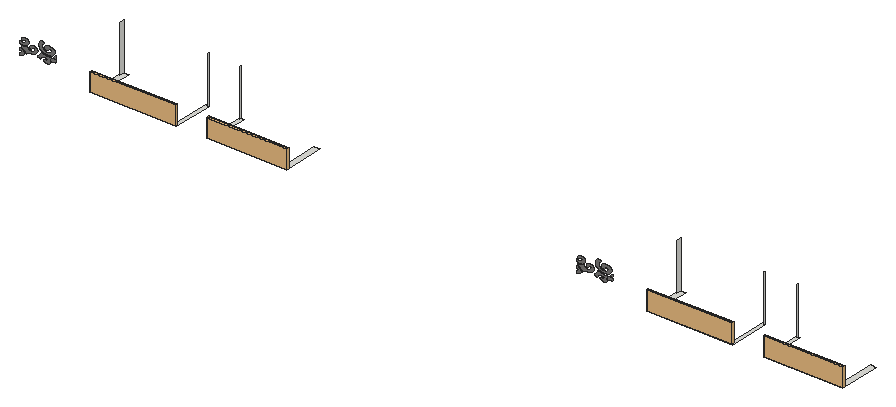
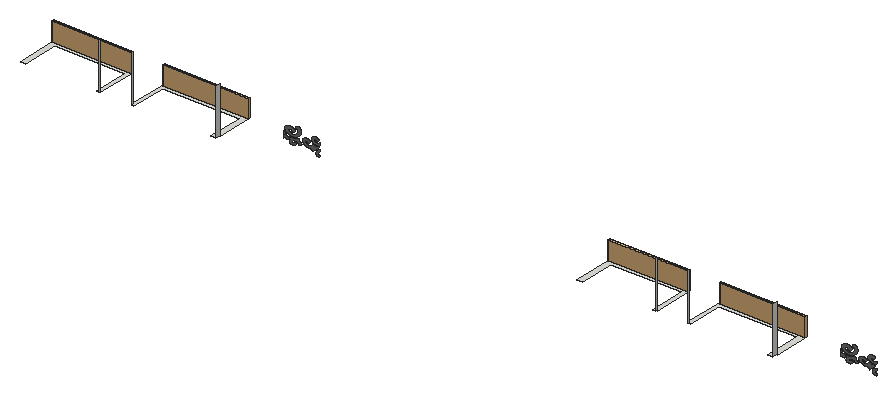
# SketchUp Ruby script. Lengths in inches.
U = 1.inch
M = Sketchup.active_model
def pt(a) = Geom::Point3d.new(a.map { |v| v * U })
def face(e, loops, mat)
  f = e.add_face(loops[0].map { |a| pt(a) })
  loops[1..].each { |l| e.add_face(l.map { |a| pt(a) }).erase! }
  f.material = f.back_material = mat if mat
  f
end
# faces: each face lists its corners as indices into pts; further lists are holes
def faces(e, pts, list, mat = nil) = list.each { |f| face(e, (f[0].is_a?(Array) ? f : [f]).map { |l| l.map { |i| pts[i] } }, mat) }
# xy, xz, yz: faces in a plane at the given z, y or x. An outline is a flat list of corners, or four numbers for a rectangle; further outlines are holes
def ring(l) = l.size == 4 ? [[l[0], l[1]], [l[2], l[1]], [l[2], l[3]], [l[0], l[3]]] : l.each_slice(2).to_a
def flat(e, list, mat, &to3) = list.each { |f| face(e, (f[0].is_a?(Array) ? f : [f]).map { |l| ring(l).map { |u, v| to3.(u, v) } }, mat) }
def xy(e, z, list, mat = nil) = flat(e, list, mat) { |x, y| [x, y, z] }
def xz(e, y, list, mat = nil) = flat(e, list, mat) { |x, z| [x, y, z] }
def yz(e, x, list, mat = nil) = flat(e, list, mat) { |y, z| [x, y, z] }
def lines(e, pts, list) = list.each { |a, b| e.add_line(pt(pts[a]), pt(pts[b])) }
# prism: a flat outline (further loops are holes) pulled along v
def prism(e, loops, v, mat = nil)
  f = face(e, loops, mat); d = Geom::Vector3d.new(v.map { |x| x * U })
  f.pushpull(f.normal.samedirection?(d) ? d.length : -d.length)
end
def box(e, o, s, mat = nil) = prism(e, [[o, [o[0] + s[0], o[1], o[2]], [o[0] + s[0], o[1] + s[1], o[2]], [o[0], o[1] + s[1], o[2]]]], [0, 0, s[2]], mat)
def at(x, y, z, deg = 0) = Geom::Transformation.translation(pt([x, y, z])) * Geom::Transformation.rotation(ORIGIN, Z_AXIS, deg.degrees)
def axes(o, x, y, z) = Geom::Transformation.new([*x, 0, *y, 0, *z, 0, *pt(o).to_a, 1])
def part(name) = M.definitions.add(name)
# library, detail: a bought-in or finely detailed component or shape, given as its bounding box
def library(name, o, s) = part(name).tap { |d| box(d.entities, o, s) }
def detail(e, o, s) = box(e.add_group.entities, o, s)
def put(e, d, t, mat = nil) = e.add_instance(d, t).tap { |i| i.material = mat if mat }
def group(e, t, mat = nil) = e.add_group.tap { |g| g.transformation = t; g.material = mat if mat }.entities
root = M.entities
M.materials.add("[0043_SaddleBrown]4").color = [124, 123, 122]
c1 = library("Glass Railing",[0,0,0],[139.5,4.76,42])
xy(root,665.9375,[[549.88,558.125,744.19,558.125,744.19,647.91,742.44,647.91,742.44,651.03,736.65,651.03,736.65,570.83,563.08,570.83,563.08,651.03,551.76,651.03,551.76,640.11,549.88,640.11],[812.81,558.125,991.94,558.125,991.94,651.03,978.86,651.03,978.86,570.83,820.97,570.83,820.97,651.03,814.68,651.03,814.68,648.85,812.81,648.85],[1800.51,558.125,1994.82,558.125,1994.82,647.91,1993.07,647.91,1993.07,651.03,1987.28,651.03,1987.28,570.83,1813.71,570.83,1813.71,651.03,1802.38,651.03,1802.38,640.11,1800.51,640.11],[2063.43,558.125,2242.56,558.125,2242.56,651.03,2229.49,651.03,2229.49,570.83,2071.59,570.83,2071.59,651.03,2065.31,651.03,2065.31,648.85,2063.43,648.85]])
xz(root,589.17,[[368.68,664.9,369.93,664.96,371.15,665.14,372.3125,665.43,373.39,665.82,374.36,666.3125,375.19,666.89,375.875,667.53,376.39,668.23,376.73,668.98,376.88,669.74,376.85,670.51,376.62,671.27,376.27,672,375.86,672.72,375.39,673.43,374.85,674.125,374.27,674.8,373.62,675.45,372.92,676.09,372.17,676.7,371.37,677.28,370.52,677.84,369.62,678.375,368.68,678.88,368.68,674.84,369.77,674.56,370.73,674.14,371.53,673.61,372.13,672.99,372.5,672.3,372.625,671.58,372.5,670.86,372.13,670.18,371.53,669.56,370.73,669.03,369.77,668.61,368.68,668.33],[1619.31,664.9,1620.56,664.96,1621.78,665.14,1622.9375,665.43,1624.01,665.82,1624.98,666.3125,1625.82,666.89,1626.5,667.53,1627.02,668.23,1627.36,668.98,1627.51,669.74,1627.47,670.51,1627.24,671.27,1626.89,672,1626.48,672.72,1626.01,673.43,1625.48,674.125,1624.89,674.8,1624.25,675.45,1623.55,676.09,1622.8,676.7,1621.99,677.28,1621.14,677.84,1620.25,678.375,1619.31,678.88,1619.31,674.84,1620.39,674.56,1621.36,674.14,1622.15,673.61,1622.75,672.99,1623.125,672.3,1623.25,671.58,1623.125,670.86,1622.75,670.18,1622.15,669.56,1621.36,669.03,1620.39,668.61,1619.31,668.33],[428.24,668.74,429.9,668.77,431.51,669,433.02,669.43,434.35,670.04,435.45,670.81,436.27,671.69,435.71,672.49,435.26,673.32,434.9375,674.17,434.74,675.03,434.66,675.91,434.71,676.78,434.89,677.64,435.1875,678.5,435.61,679.33,436.15,680.14,436.81,680.91,437.57,681.65,435.69,681.55,433.81,681.52,431.92,681.56,430.04,681.66,428.18,681.84,426.34,682.08,424.52,682.38,422.73,682.76,420.98,683.19,419.28,683.6875,417.63,684.25,416.03,684.86,415.91,683.95,415.68,683.05,415.34,682.16,414.9,681.29,414.35,680.44,413.69,679.625,412.94,678.84,412.1,678.09,411.16,677.375,410.15,676.71,409.05,676.1,407.88,675.53,408.5,675.36,409.11,675.18,409.72,674.99,410.32,674.79,410.91,674.59,411.5,674.38,412.08,674.16,412.65,673.9375,413.21,673.71,413.77,673.47,414.32,673.22,414.86,672.97,414.96,674.16,415.49,675.32,416.41,676.37,417.68,677.28,419.25,677.99,421.02,678.48,422.93,678.72,424.88,678.7,426.77,678.42,428.52,677.89,430.05,677.15,431.27,676.22,431.3,675.93,431.32,675.64,431.33,675.35,431.32,675.06,431.3,674.77,431.26,674.48,431.21,674.1875,431.15,673.9,431.07,673.61,430.98,673.33,430.87,673.05,430.75,672.77,430.16,672.61,429.53,672.51,428.88,672.47,428.24,672.5,427.61,672.59,427.01,672.74,426.45,672.95,425.96,673.21,425.54,673.51,425.2,673.85,424.96,674.22,424.82,674.61,424.41,674.5,424.02,674.375,423.64,674.24,423.27,674.08,422.93,673.92,422.59,673.74,422.28,673.55,421.99,673.34,421.72,673.13,421.47,672.9,421.25,672.67,421.05,672.43,421.64,671.47,422.53,670.61,423.6875,669.88,425.0625,669.3125,426.6,668.93],[1678.86,668.74,1680.52,668.77,1682.14,669,1683.64,669.43,1684.98,670.04,1686.07,670.81,1686.9,671.69,1686.33,672.49,1685.89,673.32,1685.5625,674.17,1685.36,675.03,1685.29,675.91,1685.34,676.78,1685.51,677.64,1685.8125,678.5,1686.24,679.33,1686.78,680.14,1687.43,680.91,1688.2,681.65,1686.32,681.55,1684.43,681.52,1682.55,681.56,1680.67,681.66,1678.81,681.84,1676.96,682.08,1675.14,682.38,1673.36,682.76,1671.61,683.19,1669.91,683.6875,1668.25,684.25,1666.66,684.86,1666.54,683.95,1666.31,683.05,1665.97,682.16,1665.52,681.29,1664.97,680.44,1664.32,679.625,1663.57,678.84,1662.72,678.09,1661.79,677.375,1660.77,676.71,1659.67,676.1,1658.51,675.53,1659.125,675.36,1659.74,675.18,1660.34,674.99,1660.94,674.79,1661.53,674.59,1662.12,674.38,1662.7,674.16,1663.27,673.9375,1663.84,673.71,1664.39,673.47,1664.94,673.22,1665.48,672.97,1665.59,674.16,1666.11,675.32,1667.04,676.37,1668.31,677.28,1669.87,677.99,1671.65,678.48,1673.56,678.72,1675.5,678.7,1677.4,678.42,1679.15,677.89,1680.67,677.15,1681.89,676.22,1681.93,675.93,1681.95,675.64,1681.96,675.35,1681.95,675.06,1681.93,674.77,1681.89,674.48,1681.84,674.1875,1681.78,673.9,1681.7,673.61,1681.5,673.05,1681.38,672.77,1680.78,672.61,1680.16,672.51,1679.51,672.47,1678.86,672.5,1678.23,672.59,1677.63,672.74,1677.08,672.95,1676.59,673.21,1676.17,673.51,1675.83,673.85,1675.59,674.22,1675.44,674.61,1675.04,674.5,1674.64,674.375,1674.26,674.24,1673.9,674.08,1673.55,673.92,1673.22,673.74,1672.91,673.55,1672.62,673.34,1672.35,673.13,1672.1,672.9,1671.875,672.67,1671.67,672.43,1672.26,671.47,1673.15,670.61,1674.3125,669.88,1675.6875,669.3125,1677.23,668.93],[382.67,672.07,383.28,672.74,383.99,673.37,384.8125,673.94,385.72,674.47,386.71,674.93,387.77,675.33,388.89,675.66,390.0625,675.92,391.27,676.11,392.51,676.22,393.75,676.25,394.99,676.2,397.41,676.55,399.7,677.15,401.77,677.98,403.58,679.02,405.07,680.24,406.1875,681.61,406.9,683.07,407.1875,684.58,407.04,686.1,406.46,687.59,405.48,688.98,404.11,690.26,402.98,690.96,401.64,691.5,400.14,691.86,398.55,692.01,396.95,691.96,395.4,691.7,393.97,691.25,392.73,690.62,391.73,689.85,391.02,688.96,390.62,688.01,390.5625,687.02,390.625,686.71,390.74,686.41,390.9,686.12,391.11,685.84,391.37,685.57,391.67,685.32,392,685.09,392.38,684.89,392.79,684.71,393.23,684.55,393.69,684.43,394.16,684.33,394.25,684.77,394.37,685.2,394.53,685.625,394.74,686.04,394.98,686.45,395.26,686.86,395.58,687.25,395.93,687.625,396.33,687.99,396.75,688.34,397.21,688.68,397.7,689,398.63,688.71,399.48,688.34,400.23,687.89,400.86,687.37,401.35,686.8,401.6875,686.2,401.875,685.57,401.9,684.92,401.76,684.29,401.47,683.67,401.02,683.09,400.4375,682.56,399.6,681.75,398.53,681.0625,397.28,680.5,395.875,680.09,394.37,679.85,392.82,679.78,391.28,679.89,389.8,680.18,388.43,680.62,387.21,681.21,386.2,681.94,385.42,682.76,385.2,682.98,385,683.2,384.81,683.43,384.63,683.66,384.46,683.9,384.31,684.14,384.17,684.38,384.04,684.625,383.92,684.87,383.82,685.12,383.73,685.37,383.66,685.625,382.97,685.06,382.16,684.55,381.27,684.11,380.29,683.74,379.24,683.45,378.14,683.24,377.01,683.11,375.86,683.07,374.72,683.125,373.59,683.26,372.5,683.48,371.46,683.79,371.67,683.52,371.87,683.25,372.03,682.98,372.17,682.69,372.29,682.4,372.37,682.11,372.43,681.82,372.46,681.53,372.47,681.23,372.44,680.93,372.39,680.64,372.3125,680.35,373.45,679.8125,374.55,679.25,375.61,678.65,376.61,678.02,377.56,677.36,378.47,676.67,379.3125,675.96,380.11,675.22,380.84,674.47,381.51,673.6875,382.12,672.89],
  [1633.29,672.07,1633.9,672.74,1634.62,673.37,1635.4375,673.94,1636.34,674.47,1637.33,674.93,1638.4,675.33,1639.52,675.66,1640.6875,675.92,1641.9,676.11,1643.13,676.22,1644.375,676.25,1645.62,676.2,1648.04,676.55,1650.32,677.15,1652.4,677.98,1654.21,679.02,1655.69,680.24,1656.8125,681.61,1657.52,683.07,1657.8125,684.58,1657.67,686.1,1657.09,687.59,1656.1,688.98,1654.73,690.26,1653.6,690.96,1652.26,691.5,1650.76,691.86,1649.18,692.01,1647.57,691.96,1646.02,691.7,1644.59,691.25,1643.35,690.62,1642.35,689.85,1641.64,688.96,1641.25,688.01,1641.1875,687.02,1641.25,686.71,1641.36,686.41,1641.52,686.12,1641.73,685.84,1641.99,685.57,1642.29,685.32,1642.63,685.09,1643.01,684.89,1643.41,684.71,1643.85,684.55,1644.31,684.43,1644.79,684.33,1644.87,684.77,1644.99,685.2,1645.16,685.625,1645.36,686.04,1645.6,686.45,1645.89,686.86,1646.2,687.25,1646.56,687.625,1646.95,687.99,1647.375,688.34,1647.83,688.68,1648.32,689,1649.26,688.71,1650.11,688.34,1650.86,687.89,1651.48,687.37,1651.97,686.8,1652.3125,686.2,1652.5,685.57,1652.52,684.92,1652.39,684.29,1652.09,683.67,1651.65,683.09,1651.0625,682.56,1650.22,681.75,1649.16,681.0625,1647.9,680.5,1646.5,680.09,1645,679.85,1643.45,679.78,1641.91,679.89,1640.43,680.18,1639.05,680.62,1637.84,681.21,1636.82,681.94,1636.04,682.76,1635.62,683.2,1635.43,683.43,1635.25,683.66,1634.93,684.14,1634.79,684.38,1634.66,684.625,1634.55,684.87,1634.45,685.12,1634.36,685.37,1634.28,685.625,1633.59,685.06,1632.79,684.55,1631.89,684.11,1630.91,683.74,1629.87,683.45,1628.77,683.24,1627.64,683.11,1626.49,683.07,1625.34,683.125,1624.21,683.26,1623.12,683.48,1622.08,683.79,1622.3,683.52,1622.49,683.25,1622.66,682.98,1622.8,682.69,1622.91,682.4,1623,682.11,1623.06,681.82,1623.09,681.53,1623.09,681.23,1623.07,680.93,1623.02,680.64,1622.9375,680.35,1624.08,679.8125,1625.18,679.25,1626.23,678.65,1627.24,678.02,1628.19,677.36,1629.09,676.67,1629.9375,675.96,1630.73,675.22,1631.46,674.47,1632.14,673.6875,1632.75,672.89],[440.77,675.97,441.32,675.99,441.78,676.05,442.23,676.14,442.67,676.25,443.09,676.38,443.49,676.54,443.87,676.72,444.21,676.91,444.53,677.13,444.82,677.36,445.07,677.61,445.29,677.87,445.46,678.14,445.81,678.02,446.15,677.9,446.48,677.77,447.12,677.49,447.42,677.34,447.72,677.18,448.01,677.02,448.29,676.85,448.5625,676.67,448.82,676.49,449.07,676.31,449.07,681.23,448.1,681.5625,447.05,681.79,445.96,681.91,444.85,681.93,443.76,681.83,442.69,681.63,441.7,681.33,440.79,680.9375,440,680.46,439.35,679.91,438.84,679.3,438.5,678.66,438.24,678.36,438.08,678.04,438.03,677.71,438.08,677.375,438.23,677.05,438.49,676.76,438.82,676.5,439.24,676.28,439.72,676.12,440.23,676.01],[1691.4,675.97,1691.94,675.99,1692.41,676.05,1692.86,676.14,1693.3,676.25,1693.72,676.38,1694.12,676.54,1694.49,676.72,1694.84,676.91,1695.16,677.13,1695.44,677.36,1695.7,677.61,1695.91,677.87,1696.09,678.14,1696.77,677.9,1697.1,677.77,1697.43,677.63,1697.74,677.49,1698.05,677.34,1698.35,677.18,1698.64,677.02,1698.92,676.85,1699.1875,676.67,1699.45,676.49,1699.7,676.31,1699.7,681.23,1698.72,681.5625,1697.68,681.79,1696.59,681.91,1695.48,681.93,1694.38,681.83,1693.32,681.63,1692.32,681.33,1691.42,680.9375,1690.63,680.46,1689.97,679.91,1689.46,679.3,1689.12,678.66,1688.87,678.36,1688.71,678.04,1688.65,677.71,1688.7,677.375,1688.86,677.05,1689.11,676.76,1689.45,676.5,1689.87,676.28,1690.34,676.12,1690.86,676.01],[448.69,684.18,449.07,684.19,449.07,689.38,448.79,689.01,448.5,688.64,448.2,688.27,447.88,687.91,447.55,687.55,447.21,687.19,446.86,686.84,446.5,686.49,446.12,686.15,445.73,685.82,445.34,685.48,444.93,685.16,445.2,685,445.5,684.85,445.81,684.71,446.13,684.59,446.47,684.48,446.83,684.39,447.1875,684.32,447.56,684.26,447.93,684.22,448.3125,684.19],[1699.32,684.18,1699.7,684.19,1699.7,689.38,1699.42,689.01,1699.125,688.64,1698.82,688.27,1698.51,687.91,1698.18,687.55,1697.84,687.19,1697.12,686.49,1696.75,686.15,1696.36,685.82,1695.96,685.48,1695.55,685.16,1695.83,685,1696.12,684.85,1696.43,684.71,1696.76,684.59,1697.1,684.48,1697.45,684.39,1697.8125,684.32,1698.18,684.26,1698.56,684.22,1698.9375,684.19],
  [430.57,686.15,432.77,686.25,434.93,686.52,437.01,686.97,438.97,687.6,440.78,688.38,442.39,689.3,443.79,690.35,444.9375,691.51,445.82,692.75,446.42,694.06,446.73,695.4,446.72,696.5625,446.4375,697.72,445.88,698.83,445.07,699.88,444.02,700.85,442.74,701.71,441.28,702.45,439.65,703.05,437.9,703.5,436.0625,703.79,434.17,703.9,432.28,703.85,430.81,703.66,429.4,703.33,428.11,702.87,426.95,702.27,425.97,701.58,425.1875,700.79,424.625,699.93,424.3,699.03,424.22,698.11,424.39,697.1875,424.79,696.3,425.43,695.47,425.95,695.13,426.56,694.86,427.26,694.68,428,694.59,428.75,694.6,429.48,694.7,430.17,694.89,430.77,695.16,431.28,695.5,431.66,695.9,431.89,696.34,431.78,696.64,431.72,696.95,431.72,697.26,431.77,697.57,431.88,697.87,432.04,698.16,432.26,698.4375,432.52,698.7,432.84,698.94,433.19,699.16,433.58,699.36,434.01,699.52,435.02,699.43,435.99,699.25,436.91,698.98,437.75,698.62,438.49,698.1875,439.12,697.69,439.61,697.14,439.96,696.56,440.16,695.94,440.21,695.3125,440.09,694.69,439.82,694.09,439.08,693.08,438.07,692.16,436.82,691.35,435.375,690.6875,433.77,690.18,432.05,689.85,430.26,689.69,428.45,689.72,426.68,689.9375,424.99,690.33,423.4375,690.89,422.05,691.6,420.6,692.61,419.38,693.73,418.41,694.93,417.7,696.2,417.27,697.52,417.125,698.87,417.27,700.21,417.7,701.53,418.41,702.8,419.38,704,420.6,705.12,422.05,706.125,421.69,706.42,421.31,706.71,420.9,706.98,420.48,707.24,420.03,707.49,419.57,707.73,419.09,707.96,418.6,708.17,418.09,708.36,417.5625,708.55,417.02,708.71,416.47,708.87,415.35,707.95,414.34,706.98,413.45,705.98,412.6875,704.93,412.05,703.85,411.55,702.75,411.18,701.625,410.95,700.49,410.85,699.34,410.9,698.19,411.08,697.05,411.4,695.92,411.93,694.7,412.66,693.52,413.59,692.4,414.69,691.33,415.97,690.34,417.4,689.4375,418.97,688.63,420.67,687.92,422.48,687.32,424.38,686.84,426.35,686.48,428.37,686.25],[1681.2,686.15,1683.4,686.25,1685.56,686.52,1687.64,686.97,1689.6,687.6,1691.4,688.38,1693.02,689.3,1694.41,690.35,1695.5625,691.51,1696.45,692.75,1697.05,694.06,1697.35,695.4,1697.35,696.5625,1697.0625,697.72,1696.51,698.83,1695.7,699.88,1694.64,700.85,1693.37,701.71,1691.9,702.45,1690.28,703.05,1688.52,703.5,1686.6875,703.79,1684.8,703.9,1682.9,703.85,1681.43,703.66,1680.03,703.33,1678.73,702.87,1677.58,702.27,1676.59,701.58,1675.8125,700.79,1675.25,699.93,1674.93,699.03,1674.84,698.11,1675.01,697.1875,1675.42,696.3,1676.06,695.47,1676.57,695.13,1677.19,694.86,1677.88,694.68,1678.62,694.59,1679.37,694.6,1680.11,694.7,1680.79,694.89,1681.4,695.16,1681.9,695.5,1682.28,695.9,1682.52,696.34,1682.4,696.64,1682.34,696.95,1682.34,697.26,1682.4,697.57,1682.5,697.87,1682.67,698.16,1682.88,698.4375,1683.15,698.7,1683.46,698.94,1683.82,699.16,1684.21,699.36,1684.63,699.52,1685.64,699.43,1686.62,699.25,1687.54,698.98,1688.38,698.62,1689.12,698.1875,1689.74,697.69,1690.24,697.14,1690.59,696.56,1690.79,695.94,1690.83,695.3125,1690.72,694.69,1690.45,694.09,1689.7,693.08,1688.69,692.16,1687.45,691.35,1686,690.6875,1684.39,690.18,1682.67,689.85,1680.89,689.69,1679.08,689.72,1677.31,689.9375,1675.62,690.33,1674.0625,690.89,1672.68,691.6,1671.23,692.61,1670.01,693.73,1669.03,694.93,1668.32,696.2,1667.9,697.52,1667.75,698.87,1667.9,700.21,1668.32,701.53,1669.03,702.8,1670.01,704,1671.23,705.12,1672.68,706.125,1672.32,706.42,1671.93,706.71,1671.53,706.98,1671.1,707.24,1670.66,707.49,1670.2,707.73,1669.72,707.96,1669.22,708.17,1668.71,708.36,1668.1875,708.55,1667.65,708.71,1667.1,708.87,1665.98,707.95,1664.97,706.98,1664.08,705.98,1663.3125,704.93,1662.68,703.85,1662.17,702.75,1661.8,701.625,1661.57,700.49,1661.48,699.34,1661.52,698.19,1661.71,697.05,1662.03,695.92,1662.56,694.7,1663.29,693.52,1664.21,692.4,1665.32,691.33,1666.59,690.34,1668.02,689.4375,1669.6,688.63,1671.3,687.92,1673.11,687.32,1675.01,686.84,1676.97,686.48,1678.99,686.25],[375.68,686.97,376.75,687.01,377.82,687.11,378.86,687.28,379.87,687.51,380.84,687.79,382.54,688.47,384.04,689.3,385.3,690.27,386.29,691.36,386.99,692.52,387.37,693.74,387.43,694.98,387.17,696.21,386.59,697.4,385.7,698.52,384.54,699.53,383.125,700.42,382.15,700.93,381.03,701.32,379.81,701.57,378.54,701.68,377.25,701.64,376.01,701.45,374.84,701.11,373.8,700.65,372.92,700.08,372.23,699.41,371.75,698.68,371.51,697.9,371.42,697.61,371.43,697.3,371.53,697,371.72,696.72,372,696.47,372.35,696.26,372.77,696.09,373.23,695.98,373.71,695.92,374.21,695.92,374.69,695.98,375.15,696.1,375.42,696.3125,375.71,696.52,376.02,696.71,376.34,696.89,376.69,697.06,377.05,697.21,377.43,697.35,377.82,697.48,378.23,697.59,378.64,697.68,379.0625,697.76,379.49,697.82,380.06,697.53,380.55,697.1875,380.98,696.82,381.33,696.42,381.6,695.99,381.78,695.55,381.88,695.1,381.88,694.64,381.79,694.1875,381.61,693.75,381.35,693.32,381,692.92,380.27,692.31,379.38,691.79,378.37,691.36,377.25,691.05,376.0625,690.86,374.84,690.8,373.62,690.86,372.43,691.05,371.3125,691.36,370.3,691.79,369.41,692.31,368.68,692.92,368.68,688.45,369.56,688.0625,370.49,687.73,371.47,687.46,372.49,687.24,373.54,687.09,374.6,687],[1626.3,686.97,1627.38,687.01,1628.44,687.11,1629.49,687.28,1630.5,687.51,1631.47,687.79,1633.16,688.47,1634.66,689.3,1635.92,690.27,1636.91,691.36,1637.61,692.52,1637.99,693.74,1638.06,694.98,1637.79,696.21,1637.21,697.4,1636.33,698.52,1635.16,699.53,1633.75,700.42,1632.77,700.93,1631.65,701.32,1630.43,701.57,1629.16,701.68,1627.88,701.64,1626.63,701.45,1625.47,701.11,1624.42,700.65,1623.54,700.08,1622.85,699.41,1622.375,698.68,1622.14,697.9,1622.05,697.61,1622.05,697.3,1622.15,697,1622.35,696.72,1622.625,696.47,1622.98,696.26,1623.39,696.09,1623.85,695.98,1624.34,695.92,1624.83,695.92,1625.32,695.98,1625.78,696.1,1626.04,696.3125,1626.33,696.52,1626.64,696.71,1626.97,696.89,1627.32,697.06,1627.68,697.21,1628.06,697.35,1628.45,697.48,1628.85,697.59,1629.26,697.68,1629.6875,697.76,1630.12,697.82,1630.68,697.53,1631.18,697.1875,1631.61,696.82,1631.96,696.42,1632.23,695.99,1632.41,695.55,1632.5,695.1,1632.5,694.64,1632.41,694.1875,1632.24,693.75,1631.97,693.32,1631.62,692.92,1630.89,692.31,1630.01,691.79,1628.99,691.36,1627.875,691.05,1626.6875,690.86,1625.46,690.8,1624.24,690.86,1623.05,691.05,1621.9375,691.36,1620.92,691.79,1620.04,692.31,1619.31,692.92,1619.31,688.45,1620.18,688.0625,1621.11,687.73,1622.09,687.46,1623.11,687.24,1624.16,687.09,1625.23,687]],"[0043_SaddleBrown]4")
xz(root,651.03,[[814.68,665.9375,814.89,771.4375],[2065.31,665.9375,2065.52,771.4375]])
yz(root,551.76,[[640.11,665.9375,651.03,771.4375]])
yz(root,742.44,[[647.91,665.9375,651.03,771.4375]])
yz(root,814.68,[[648.85,665.9375,651.03,771.4375]])
yz(root,1802.38,[[640.11,665.9375,651.03,771.4375]])
yz(root,1993.07,[[647.91,665.9375,651.03,771.4375]])
yz(root,2065.31,[[648.85,665.9375,651.03,771.4375]])
put(root,c1,axes([549.88,558.125,665.9375],[1.37946,0,0],[0,1,0],[0,0,1]))
put(root,c1,axes([812.81,558.125,665.9375],[1.28407,0,0],[0,1,0],[0,0,1]))
put(root,c1,axes([1800.51,558.125,665.9375],[1.37946,0,0],[0,1,0],[0,0,1]))
put(root,c1,axes([2063.43,558.125,665.9375],[1.28407,0,0],[0,1,0],[0,0,1]))
